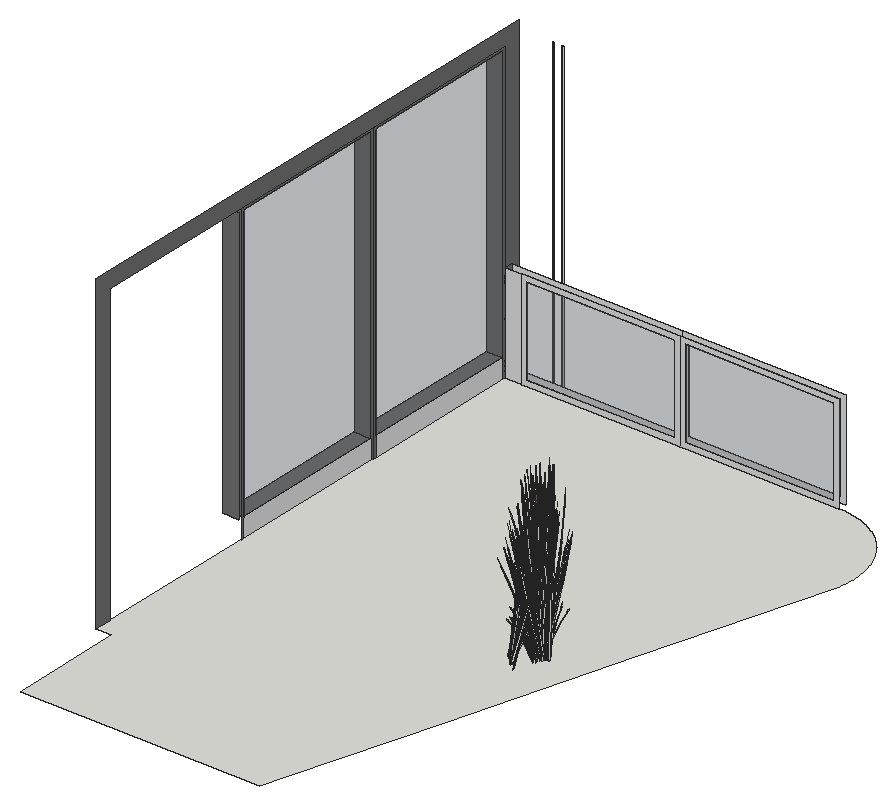
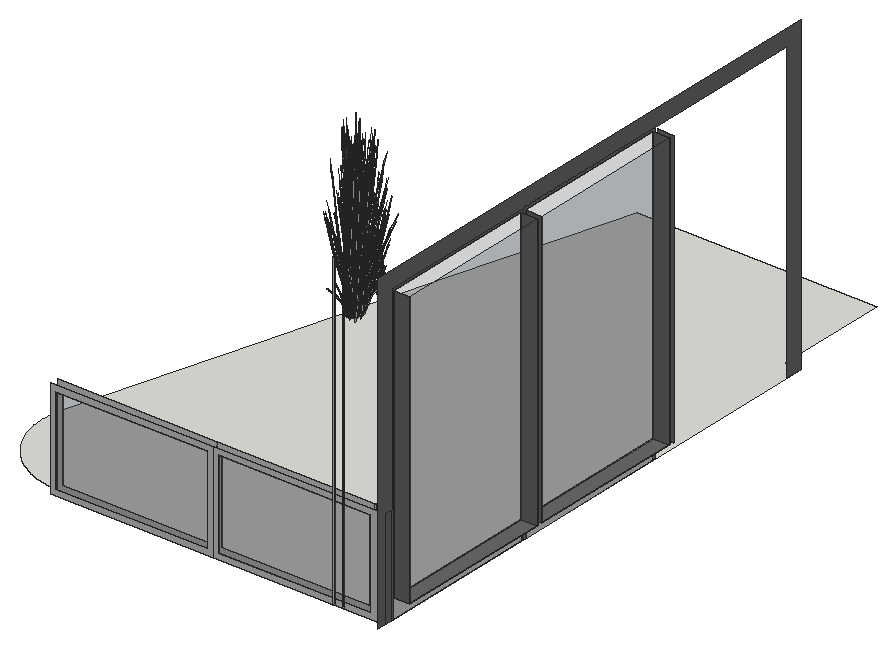
# SketchUp Ruby script. Lengths in inches.
U = 1.inch
M = Sketchup.active_model
def pt(a) = Geom::Point3d.new(a.map { |v| v * U })
def face(e, loops, mat)
  f = e.add_face(loops[0].map { |a| pt(a) })
  loops[1..].each { |l| e.add_face(l.map { |a| pt(a) }).erase! }
  f.material = f.back_material = mat if mat
  f
end
# faces: each face lists its corners as indices into pts; further lists are holes
def faces(e, pts, list, mat = nil) = list.each { |f| face(e, (f[0].is_a?(Array) ? f : [f]).map { |l| l.map { |i| pts[i] } }, mat) }
# xy, xz, yz: faces in a plane at the given z, y or x. An outline is a flat list of corners, or four numbers for a rectangle; further outlines are holes
def ring(l) = l.size == 4 ? [[l[0], l[1]], [l[2], l[1]], [l[2], l[3]], [l[0], l[3]]] : l.each_slice(2).to_a
def flat(e, list, mat, &to3) = list.each { |f| face(e, (f[0].is_a?(Array) ? f : [f]).map { |l| ring(l).map { |u, v| to3.(u, v) } }, mat) }
def xy(e, z, list, mat = nil) = flat(e, list, mat) { |x, y| [x, y, z] }
def xz(e, y, list, mat = nil) = flat(e, list, mat) { |x, z| [x, y, z] }
def yz(e, x, list, mat = nil) = flat(e, list, mat) { |y, z| [x, y, z] }
def lines(e, pts, list) = list.each { |a, b| e.add_line(pt(pts[a]), pt(pts[b])) }
# prism: a flat outline (further loops are holes) pulled along v
def prism(e, loops, v, mat = nil)
  f = face(e, loops, mat); d = Geom::Vector3d.new(v.map { |x| x * U })
  f.pushpull(f.normal.samedirection?(d) ? d.length : -d.length)
end
def box(e, o, s, mat = nil) = prism(e, [[o, [o[0] + s[0], o[1], o[2]], [o[0] + s[0], o[1] + s[1], o[2]], [o[0], o[1] + s[1], o[2]]]], [0, 0, s[2]], mat)
def at(x, y, z, deg = 0) = Geom::Transformation.translation(pt([x, y, z])) * Geom::Transformation.rotation(ORIGIN, Z_AXIS, deg.degrees)
def axes(o, x, y, z) = Geom::Transformation.new([*x, 0, *y, 0, *z, 0, *pt(o).to_a, 1])
def part(name) = M.definitions.add(name)
# library, detail: a bought-in or finely detailed component or shape, given as its bounding box
def library(name, o, s) = part(name).tap { |d| box(d.entities, o, s) }
def detail(e, o, s) = box(e.add_group.entities, o, s)
def put(e, d, t, mat = nil) = e.add_instance(d, t).tap { |i| i.material = mat if mat }
def group(e, t, mat = nil) = e.add_group.tap { |g| g.transformation = t; g.material = mat if mat }.entities
root = M.entities
M.materials.add("Glass_Basic_01").color = [105, 113, 122]
M.materials["Glass_Basic_01"].alpha = 0.25
M.materials.add("LightPink_Translucent").color = [144, 107, 117]
M.materials["LightPink_Translucent"].alpha = 0.75
M.materials.add("M01_Silver_Fog").color = [224, 224, 224]
M.materials.add("M06_Steel_Smoke").color = [114, 114, 114]
c1 = part("blade")
p = [[2.15,0.21,22],[0,0.17,0],[0.09,0.45,0],[2.18,0.31,22],[2.29,0.31,22],[0.38,0.45,0],
  [2.48,0.24,33],[2.49,0.24,33],[2.48,0.22,33]]
faces(c1.entities,p,[[0,1,2,3],[4,5,2,3],[6,3,4,7],[8,0,3,6]])
c2 = part("seeds")
p = [[0.3,-0.1,1.38],[-0.01,-0.03,1.59],[-0.01,-0.03,0.03],[0.14,-0.07,-0.07],[0.29,-0.03,3],[0.15,0.01,3.11]]
faces(c2.entities,p,[[0,1,2,3],[1,0,4,5]],"LightPink_Translucent")
c3 = part("blade with seeds")
put(c3.entities,c1,at(0,0,0))
put(c3.entities,c2,axes([2.4,0.25,30.99],[1.5799,-0.05474,1.17369],[-0.12525,1.92788,0.29478],[-0.07173,-0.02425,1.56792]))
xy(root,270,[[216,246,303.26,246,306,255.36,321.22,307.35,340.07,371.78,359.17,437.01,359.4,437.91,359.63,439,359.83,440.1,359.98,441.21,360.09,442.32,360.16,443.43,360.1875,444.55,360.17,445.67,360.11,446.78,360.01,447.89,359.87,449,359.68,450.1,359.45,451.2,359.18,452.28,358.875,453.35,358.52,454.41,358.13,455.46,357.7,456.49,357.23,457.5,356.73,458.5,356.18,459.47,355.6,460.43,354.98,461.36,354.33,462.26,353.64,463.14,352.92,464,352.17,464.83,351.39,465.62,350.58,466.39,349.74,467.125,348.87,467.83,347.97,468.5,347.05,469.13,346.11,469.73,345.15,470.29,344.16,470.82,343.16,471.3,342.13,471.75,341.09,472.16,340.04,472.53,338.97,472.86,337.89,473.15,336.8,473.4,335.71,473.6,334.6,473.77,333.49,473.89,332.38,473.97,331.45,474,210,474,210,288,213,288,213,287.79,216,287.79]])
xy(root,277,[[204,355,210,413],[204,415,210,473]],"M06_Steel_Smoke")
xz(root,353,[[204,277,210,377]],"M06_Steel_Smoke")
xz(root,355,[[204,277,210,377]],"M06_Steel_Smoke")
xz(root,413,[[204,277,210,377]],"M06_Steel_Smoke")
xz(root,415,[[204,277,210,377]],"M06_Steel_Smoke")
xz(root,473,[[204,277,210,377]],"M06_Steel_Smoke")
xz(root,474,[[218,272,271.49,304],[275.49,272,329.45,304]],"Glass_Basic_01")
xz(root,474,[[210,270,215.53,306],[215.53,270,216,306],[[216,270,273.49,306],[218,272,271.49,304]],[[273.49,270,331.45,306],[275.49,272,329.45,304]]],"M01_Silver_Fog")
xz(root,477,[[215,272,270.25,304],[274.25,272,329.5,304]],"Glass_Basic_01")
xz(root,477,[[[210,270,272.25,306],[215,272,270.25,304]],[[272.25,270,331.5,306],[274.25,272,329.5,304]]],"M01_Silver_Fog")
xz(root,477.03,[[225.03,270,225.12,383.24],[225.12,270,225.2,383.24],[225.2,270,225.29,383.24],[228.34,270,228.43,383.24],[228.43,270,228.52,383.24],
  [228.52,270,228.6,383.24]],"M01_Silver_Fog")
yz(root,204,[[355,277,413,377],[415,277,473,377]],"Glass_Basic_01")
yz(root,210,[[355,277,413,377],[415,277,473,377]],"Glass_Basic_01")
yz(root,210,[[355,270,413,277],[415,270,473,277]],"M01_Silver_Fog")
yz(root,210,[[288,270,294,270,294,378,474,378,474,306,477,306,477,270,480,270,480,384,288,384],[354,270,355,270,355,377,413,377,413,270,414,270,414,378,354,378],[414,270,415,270,415,377,473,377,473,270,474,270,474,378,414,378],[474,270,477,306]],"M06_Steel_Smoke")
p = [[224.94,477.04,270],[225.03,477.03,270],[225.03,477.03,383.24],[224.94,477.04,383.24],[224.85,477.06,270],[224.85,477.06,383.24],
  [225.29,477.03,270],[225.38,477.04,270],[225.38,477.04,383.24],[225.29,477.03,383.24],[228.17,477.06,270],[228.25,477.04,270],
  [228.25,477.04,383.24],[228.17,477.06,383.24],[228.34,477.03,270],[228.34,477.03,383.24],[228.6,477.03,270],[228.69,477.04,270],
  [228.69,477.04,383.24],[228.6,477.03,383.24]]
faces(root,p,[[0,1,2,3],[4,0,3,5],[6,7,8,9],[10,11,12,13],[11,14,15,12],[16,17,18,19]],"M01_Silver_Fog")
put(root,c3,axes([325.15,344.34,274.77],[0.06446,0.31404,1.1486],[-0.35756,-0.17393,0.84392],[0.03848,-0.1608,0.25299]))
put(root,c3,axes([320.96,338.65,273.49],[0.08132,-0.0293,1.76342],[0.48914,0.1613,-0.26939],[0.0143,0.18179,0.30037]))
put(root,c3,axes([323.96,344.07,276.71],[-0.00937,0.06455,1.77383],[-0.46231,0.23427,-0.16761],[-0.13604,-0.11975,0.31391]))
put(root,c3,axes([320.23,338.18,277],[0.35968,0.36185,-0.5672],[-0.37996,0.3169,-0.43934],[-0.05473,0.18385,1.08528]))
put(root,c3,axes([319.84,338.72,274.82],[0.45645,-0.09537,0.06507],[0.10494,0.38421,-0.86304],[-0.02894,0.19449,0.7736]))
put(root,c3,axes([321.3,338.53,276.68],[0.49392,0.135,-0.51099],[-0.1693,0.46287,-0.3958],[0.04529,0.18636,0.97773]))
put(root,c3,axes([321.58,337.57,275.875],[-0.11485,-0.17291,1.71376],[0.53072,-0.14557,0.13857],[0.11995,0.27145,0.73262]))
put(root,c3,axes([323.86,345.21,277.09],[0.55971,-0.13842,0.53763],[0.09714,0.54299,0.4433],[-0.13164,-0.16003,1.11249]))
put(root,c3,axes([325.13,345.3125,276.73],[0.4951,0.14079,0.48003],[-0.1693,0.46287,0.3958],[-0.02975,-0.18203,0.9933]))
put(root,c3,axes([325.27,345.48,277.03],[-0.49168,0.25073,-0.1216],[-0.24162,-0.44501,-0.67495],[-0.06487,-0.18753,1.02557]))
put(root,c3,axes([326.29,346.04,277.03],[-0.55221,-0.02668,-0.1216],[0.01509,-0.50521,-0.67495],[0.03836,-0.19458,1.02557]))
put(root,c3,axes([323.31,344.72,274.77],[0.2621,0.18744,1.1486],[-0.38171,0.11267,0.84392],[-0.08167,-0.14405,0.25299]))
put(root,c3,axes([321.07,338.8125,276.53],[-0.15148,0.41415,-0.35414],[-0.44193,-0.12079,0.4572],[0.04052,0.16674,0.87481]))
put(root,c3,axes([325.26,345.28,276.73],[0.37023,-0.18303,0.0643],[0.18122,0.33376,0.50621],[-0.03575,-0.14712,0.77189]))
put(root,c3,axes([323.95,345.71,276.98],[-0.42844,-0.2603,-0.71045],[0.30448,-0.45614,0.08574],[-0.15523,-0.15542,1.00501]))
put(root,c3,axes([323.8,345.37,276.53],[-0.0776,-0.43378,-0.35414],[0.44361,-0.11454,0.4572],[-0.11915,-0.12431,0.87481]))
put(root,c3,axes([320.12,338.01,277.34],[-0.01307,0.49815,-0.7886],[-0.55054,-0.03346,0.09517],[-0.0581,0.21104,1.11556]))
put(root,c3,axes([318.68,339.32,276.71],[0.057,-0.03251,1.77383],[0.47114,0.21627,-0.16761],[-0.01107,0.18007,0.31391]))
put(root,c3,axes([320.64,337.66,275.875],[-0.0123,-0.2067,1.71376],[0.53301,0.13712,0.13857],[-0.03297,0.29456,0.73262]))
put(root,c3,axes([323.99,345.33,276.73],[0.22836,-0.34211,0.0643],[0.3252,0.19918,0.50621],[-0.10513,-0.10968,0.77189]))
put(root,c3,axes([323.11,345.28,273.49],[-0.04867,0.07094,1.76342],[-0.49185,0.15296,-0.26939],[-0.11882,-0.13915,0.30037]))
put(root,c3,axes([321.12,338.44,276.98],[0.23981,0.43789,-0.71045],[-0.49365,0.24404,0.08574],[0.05608,0.21158,1.00501]))
put(root,c3,axes([323.92,347.23,274.1],[-0.20635,-0.55225,-0.69835],[0.59439,-0.19889,-0.18329],[-0.02281,-0.18701,1.54149]))
put(root,c3,axes([322.84,346,275.875],[0.18664,0.09279,1.71376],[-0.38624,0.38925,0.13857],[-0.24072,-0.1756,0.73262]))
put(root,c3,axes([319.73,339.13,274.59],[0.15856,-0.08496,1.43002],[0.39147,0.25616,-0.30754],[-0.11652,0.22165,0.61141]))
put(root,c3,axes([320.76,339.55,276.72],[0.06369,0.08672,1.74944],[0.51399,0.03407,-0.27667],[0.05169,0.19126,0.14031]))
put(root,c3,axes([325.12,345.65,277.05],[-0.15148,0.41415,0.35414],[-0.44193,-0.12079,-0.4572],[-0.04052,-0.16674,0.87481]))
put(root,c3,axes([323.75,345.73,276.68],[-0.4958,0.12802,-0.51099],[-0.08673,-0.48481,-0.3958],[-0.13317,-0.13893,0.97773]))
put(root,c3,axes([324.09,345.29,277.43],[-0.33533,0.51628,-0.13619],[-0.48563,-0.29744,-0.75594],[-0.16881,-0.14586,1.14864]))
put(root,c3,axes([323.84,345.65,274.375],[-0.31414,-0.53965,0],[0.52557,-0.30095,-0.51607],[0.1197,-0.06854,1.63711]))
put(root,c3,axes([324.53,345,274.13],[-0.34721,0.30895,-0.03893],[-0.31814,-0.33837,-0.17649],[-0.0224,-0.09588,0.58215]))
put(root,c3,axes([319.93,338.71,275.36],[0.01104,-0.27801,1.54345],[0.49652,0.14685,0.21329],[-0.04302,0.2963,0.72882]))
put(root,c3,axes([322.81,345.14,276.72],[-0.10811,-0.0038,1.74944],[-0.34418,0.38014,-0.27667],[-0.18364,-0.07767,0.14031]))
put(root,c3,axes([324.97,348.66,275.33],[0.4342,0.21716,1.51261],[-0.42537,0.46784,0.59816],[-0.19053,-0.27728,1.26806]))
put(root,c3,axes([324.0625,345.72,277.05],[0.0776,0.43378,0.35414],[-0.44361,0.11454,-0.4572],[-0.11915,-0.12431,0.87481]))
put(root,c3,axes([322.7,347.16,274.02],[0,-0.53854,-0.49651],[0.56215,0,0],[0,-0.12266,1.57504]))
put(root,c3,axes([322.73,346,277.09],[0.41494,-0.39744,0.53763],[0.35786,0.42207,0.4433],[-0.19468,-0.07331,1.11249]))
put(root,c3,axes([322.92,346,276.73],[0.0253,-0.40952,0.0643],[0.38204,0.01123,0.50621],[-0.14634,-0.04285,0.77189]))
put(root,c3,axes([324.23,347.375,274.21],[0.24378,-0.48527,-0.44739],[0.50654,0.23354,0.21531],[0,-0.11186,1.43643]))
put(root,c3,axes([322.77,346.13,276.53],[-0.28589,-0.33718,-0.35414],[0.32644,-0.31919,0.4572],[-0.16586,-0.04856,0.87481]))
put(root,c3,axes([322.94,347.17,274.03],[0.35073,-0.33601,-0.30978],[0.35073,0.33601,0.30978],[0,-0.10823,1.38974]))
put(root,c3,axes([322.8,345.56,274.13],[-0.14494,0.43975,-0.03893],[-0.4461,-0.13527,-0.17649],[-0.06773,-0.07192,0.58215]))
put(root,c3,axes([324.17,347.78,274.67],[-0.56585,-0.25696,-0.29095],[0.27246,-0.54236,-0.50002],[-0.01778,-0.13316,1.59708]))
put(root,c3,axes([322.5625,347.56,274.375],[-0.62828,0,0],[0,-0.6019,-0.51607],[0,-0.13709,1.63711]))
put(root,c3,axes([322.67,346.49,274.59],[0.0981,0.14994,1.43002],[-0.22605,0.40756,-0.30754],[-0.23211,-0.09741,0.61141]))
put(root,c3,axes([323.07,346.36,276.98],[-0.50227,-0.01297,-0.71045],[0.03373,-0.54602,0.08574],[-0.21278,-0.05762,1.00501]))
put(root,c3,axes([323.05,347.41,274.33],[-0.46736,0.45277,0.30756],[-0.46764,-0.44801,-0.36492],[-0.01632,-0.12858,1.64885]))
put(root,c3,axes([322.39,345.47,276.71],[0.03725,0.05374,1.77383],[-0.17957,0.48312,-0.16761],[-0.18186,0.0035,0.31391]))
put(root,c3,axes([324.53,347.62,274.43],[0.56613,0.26102,0.24065],[-0.27246,0.54236,0.50002],[0,-0.12502,1.60543]))
put(root,c3,axes([324.3125,348.35,274.4375],[0.13317,-0.63814,-0.23429],[0.63143,0.11124,0.51271],[-0.11033,-0.08813,1.5644]))
put(root,c3,axes([322.91,346.47,276.68],[-0.36484,0.35674,-0.51099],[-0.31952,-0.37685,-0.3958],[-0.18537,-0.05428,0.97773]))
put(root,c3,axes([323.18,346.31,277.05],[0.28589,0.33718,0.35414],[-0.32644,0.31919,-0.4572],[-0.16586,-0.04856,0.87481]))
put(root,c3,axes([322.09,346.9375,274.77],[0.32078,-0.03854,1.1486],[-0.20348,0.33954,0.84392],[-0.15852,-0.05093,0.25299]))
put(root,c3,axes([324.35,347.25,274.72],[-0.54562,0.03324,0.44739],[-0.04934,-0.55185,-0.21531],[0.09768,-0.05593,1.43643]))
put(root,c3,axes([323.1,346.09,277.03],[-0.0269,0.54769,-0.1216],[-0.50939,-0.01497,-0.67495],[-0.19618,-0.03804,1.02557]))
put(root,c3,axes([322.94,347.66,274.48],[0,0.53854,0.49651],[-0.56215,0,0],[0,-0.12266,1.57504]))
put(root,c3,axes([322.45,346.85,275.875],[0.20841,-0.0122,1.71376],[-0.13825,0.52864,0.13857],[-0.297,-0.0327,0.73262]))
put(root,c3,axes([324.27,348.09,274.21],[-0.30184,-0.45202,-0.44739],[0.45719,-0.31831,0.21531],[-0.09768,-0.05593,1.43643]))
put(root,c3,axes([324.33,347.45,274.36],[0.21845,0.6022,0.45755],[-0.62418,0.20941,0.17955],[0.00763,-0.11065,1.58856]))
put(root,c3,axes([324.22,347.93,274.72],[-0.24378,0.48527,0.44739],[-0.50654,-0.23354,-0.21531],[0,-0.11186,1.43643]))
put(root,c3,axes([325.12,347.5,274.21],[0,-0.62313,0],[0.62828,0,0],[0,0,1.79456]))
put(root,c3,axes([324,348.26,274.06],[-0.52267,-0.08829,-0.62353],[0.11029,-0.54463,-0.16365],[-0.15598,-0.06599,1.37633]))
put(root,c3,axes([324.82,347.11,274.36],[-0.4166,0.48873,0.45755],[-0.49494,-0.43142,0.17955],[0.10044,-0.04877,1.58856]))
put(root,c3,axes([325.28,347.99,274.3],[-0.46736,-0.46353,-0.06131],[0.46764,-0.46381,0],[-0.01632,-0.01619,1.75571]))
put(root,c3,axes([324.1,346.31,274.47],[-0.14515,0.53522,0.17642],[-0.53115,-0.15146,0.35086],[0.09175,-0.00261,1.60407]))
put(root,c3,axes([322.36,347.25,276.73],[0.14195,-0.49104,0.48003],[0.46669,0.16791,0.3958],[-0.18353,0.02951,0.9933]))
put(root,c3,axes([322.33,347.12,276.73],[-0.18454,-0.3672,0.0643],[0.33652,-0.17973,0.50621],[-0.14834,0.03546,0.77189]))
put(root,c3,axes([324.39,348.04,274.36],[0.63506,0.11347,0.45755],[-0.12924,0.64083,0.17955],[-0.09281,-0.06188,1.58856]))
put(root,c3,axes([322.32,347.49,273.49],[0.01274,0.08487,1.76342],[-0.25688,0.44323,-0.26939],[-0.18246,-0.02234,0.30037]))
put(root,c3,axes([323.44,349.09,274.03],[-0.11803,-0.46926,-0.30978],[0.46876,-0.13325,0.30978],[-0.0945,-0.05411,1.38974]))
put(root,c3,axes([324.05,349.07,274.47],[0.53992,-0.14294,0.17642],[0.13332,0.53195,0.35086],[-0.04815,-0.07751,1.60407]))
put(root,c3,axes([323.3125,349.29,274.02],[-0.47024,-0.26927,-0.49651],[0.28107,-0.48284,0],[-0.1071,-0.06133,1.57504]))
put(root,c3,axes([322.27,347.3,276.53],[-0.41757,-0.15024,-0.35414],[0.12179,-0.4383,0.4572],[-0.16812,0.04019,0.87481]))
put(root,c3,axes([324.59,348.34,274.67],[-0.5073,0.35754,-0.29095],[-0.33735,-0.5052,-0.50002],[-0.12516,-0.05131,1.59708]))
put(root,c3,axes([325.7,346.34,274.47],[-0.53992,0.14294,0.17642],[-0.13332,-0.53195,0.35086],[0.04815,0.07751,1.60407]))
put(root,c3,axes([325.36,347.36,274.38],[-0.63506,-0.11347,0.49198],[0.12924,-0.64083,0.19306],[0.09281,0.06188,1.70813]))
put(root,c3,axes([324.86,348.94,274.2],[-0.16394,-0.4643,0],[0.46814,-0.1626,0],[0,0,1.54371]))
put(root,c3,axes([324.54,348.5,274.62],[-0.09693,0.48062,0.1448],[-0.47357,-0.08343,-0.41347],[-0.08619,-0.04935,1.26744]))
put(root,c3,axes([322.71,347.25,277.05],[0.41757,0.15024,0.35414],[-0.12179,0.4383,-0.4572],[-0.16812,0.04019,0.87481]))
put(root,c3,axes([325.65,349.1,274.47],[0.14515,-0.53522,0.17642],[0.53115,0.15146,0.35086],[-0.09175,0.00261,1.60407]))
put(root,c3,axes([325.53,347.88,274.21],[0.35073,0.34786,0],[-0.35073,0.34786,0],[0,0,1.69266]))
put(root,c3,axes([323.54,347.23,275.34],[0.14282,-0.0779,1.77064],[0.04925,0.54394,0.13857],[-0.30935,0.07218,0.63284]))
put(root,c3,axes([326.48,347.73,274.47],[-0.39477,-0.39228,0.17642],[0.39783,-0.38049,0.35086],[-0.0436,0.08011,1.60407]))
put(root,c3,axes([324.74,349.15,274.2],[-0.50654,-0.24178,0],[0.24378,-0.50239,0],[0,0,1.62707]))
put(root,c3,axes([325.16,348.51,274.46],[-0.49063,-0.43346,-0.25192],[0.41285,-0.48673,0.5513],[-0.13212,0.05071,1.68216]))
put(root,c3,axes([323.87,349.34,274.48],[0.47024,0.26927,0.49651],[-0.28107,0.48284,0],[-0.1071,-0.06133,1.57504]))
put(root,c3,axes([325.53,347.47,274.72],[0.24378,-0.48527,0.44739],[0.50654,0.23354,-0.21531],[0,0.11186,1.43643]))
put(root,c3,axes([322,347.59,276.72],[-0.08205,0.06992,1.74944],[0.00698,0.51086,-0.27667],[-0.18807,0.06644,0.14031]))
put(root,c3,axes([325.43,347.75,274.29],[0,0.62282,-0.05637],[-0.62828,0,0],[0,0.01957,1.79368]))
put(root,c3,axes([322.55,347.52,276.68],[-0.13612,0.48987,-0.51099],[-0.46669,-0.16791,-0.3958],[-0.1879,0.04492,0.97773]))
put(root,c3,axes([322.53,347.11,277.03],[0.25281,0.48765,-0.1216],[-0.44869,0.23964,-0.67495],[-0.18908,0.06434,1.02557]))
put(root,c3,axes([323.6,349.62,274.375],[-0.31414,0.53965,0],[-0.52557,-0.30095,-0.51607],[-0.1197,-0.06854,1.63711]))
put(root,c3,axes([325.4,348.15,274.72],[0.54562,-0.03324,0.44739],[0.04934,0.55185,-0.21531],[-0.09768,0.05593,1.43643]))
put(root,c3,axes([324.91,348.42,274.21],[-0.54562,0.03324,-0.44739],[-0.04934,-0.55185,0.21531],[-0.09768,0.05593,1.43643]))
put(root,c3,axes([325.32,349.16,274.2],[0.50654,0.24178,0],[-0.24378,0.50239,0],[0,0,1.74954]))
put(root,c3,axes([325.52,349.69,274.19],[-0.31023,-0.54153,-0.05142],[0.52557,-0.30095,0.51607],[-0.12951,0.05156,1.6363]))
put(root,c3,axes([325.41,348.39,274.62],[0.37121,0.32357,0.1448],[-0.30963,0.36505,-0.41347],[-0.08619,0.04935,1.26744]))
put(root,c3,axes([322.48,348.47,276.73],[-0.12461,-0.49565,0.48003],[0.48882,-0.08602,0.3958],[-0.14406,0.11657,0.9933]))
put(root,c3,axes([322.38,348.375,276.73],[-0.34493,-0.22649,0.0643],[0.20082,-0.32253,0.50621],[-0.11059,0.10427,0.77189]))
put(root,c3,axes([322.54,347.78,275.875],[0.17434,-0.11391,1.71376],[0.14677,0.52637,0.13857],[-0.27369,0.11897,0.73262]))
put(root,c3,axes([325.8,349.38,274.48],[0.47024,-0.26927,0.49651],[0.28107,0.48284,0],[-0.1071,0.06133,1.57504]))
put(root,c3,axes([325.13,348.96,274.29],[0.21845,0.61869,-0.06012],[-0.62418,0.21679,0],[0.00763,0.02161,1.72173]))
put(root,c3,axes([325.375,349.625,274.03],[-0.46876,-0.13325,-0.30978],[0.11803,-0.46926,0.30978],[-0.0945,0.05411,1.38974]))
put(root,c3,axes([321.99,348.67,274.59],[0.17462,0.04421,1.43002],[0.11254,0.45156,-0.30754],[-0.23719,0.08453,0.61141]))
put(root,c3,axes([322.78,348.31,277.05],[0.43736,-0.07697,0.35414],[0.11549,0.43998,-0.4572],[-0.12533,0.11818,0.87481]))
put(root,c3,axes([321.09,348.11,276.71],[0.06412,0.01444,1.77383],[0.19837,0.47583,-0.16761],[-0.13126,0.12489,0.31391]))
put(root,c3,axes([326.9375,348.15,274.2],[-0.62797,-0.00431,-0.04976],[0,-0.6019,0.49943],[-0.01973,0.13702,1.58352]))
put(root,c3,axes([321.63,349.62,274.77],[0.2094,-0.24408,1.1486],[0.08263,0.38639,0.84392],[-0.15132,0.06919,0.25299]))
put(root,c3,axes([326.81,348.23,274.03],[-0.35073,0.33601,-0.30978],[-0.35073,-0.33601,0.30978],[0,0.10823,1.38974]))
put(root,c3,axes([325.3,348.27,274.67],[0.05855,0.61451,-0.29095],[-0.60981,0.03716,-0.50002],[-0.10738,0.08185,1.59708]))
put(root,c3,axes([325.52,348.03,274.21],[-0.24378,0.48527,-0.44739],[-0.50654,-0.23354,0.21531],[0,0.11186,1.43643]))
put(root,c3,axes([322.42,348.57,276.53],[-0.43736,0.07697,-0.35414],[-0.11549,-0.43998,0.4572],[-0.12533,0.11818,0.87481]))
put(root,c3,axes([321.78,349.55,277.65],[0.44338,0.14375,-0.06488],[-0.13639,0.44245,-0.29416],[-0.07252,0.06718,0.97024]))
put(root,c3,axes([324.93,348.73,274.06],[-0.33843,0.40479,-0.62353],[-0.42041,-0.36705,-0.16365],[-0.13561,0.10098,1.37633]))
put(root,c3,axes([325.53,349.42,274.33],[0.62903,0.17504,0.30756],[-0.15737,0.62568,-0.36492],[-0.10411,0.07831,1.64885]))
put(root,c3,axes([325.49,349.84,274.02],[-0.47024,0.26927,-0.49651],[-0.28107,-0.48284,0],[-0.1071,0.06133,1.57504]))
put(root,c3,axes([322.55,348.26,277.03],[0.46478,0.29695,-0.1216],[-0.26776,0.43004,-0.67495],[-0.13131,0.14949,1.02557]))
put(root,c3,axes([323.18,348.13,275.875],[0.1255,-0.16547,1.71376],[0.31687,0.44665,0.13857],[-0.21734,0.2034,0.73262]))
put(root,c3,axes([322.78,348.62,276.68],[0.12908,0.49174,-0.51099],[-0.48882,0.08602,-0.3958],[-0.14008,0.13208,0.97773]))
put(root,c3,axes([323.37,349.18,277.05],[0.33997,-0.28354,0.35414],[0.32182,0.32376,-0.4572],[-0.04897,0.1645,0.87481]))
put(root,c3,axes([325.91,349.76,274.375],[0.31414,0.53965,0],[-0.52557,0.30095,-0.51607],[-0.1197,0.06854,1.63711]))
put(root,c3,axes([325.65,347.62,274.84],[-0.01373,-0.50706,1.41272],[0.62119,0.13144,0.59816],[-0.14692,0.27746,1.3335]))
put(root,c3,axes([325.81,348.17,274.09],[0.18424,0.49308,-0.69212],[-0.53071,0.17758,-0.18165],[0.02036,0.16697,1.52773]))
put(root,c3,axes([323.06,349.4375,276.73],[-0.4129,-0.02509,0.0643],[0.01132,-0.37891,0.50621],[-0.04321,0.14514,0.77189]))
put(root,c3,axes([322.18,349.87,273.49],[0.0674,0.0538,1.76342],[0.11428,0.49852,-0.26939],[-0.14937,0.10631,0.30037]))
put(root,c3,axes([323.19,349.47,276.73],[-0.35779,-0.36745,0.48003],[0.37996,-0.3169,0.3958],[-0.066,0.17239,0.9933]))
put(root,c3,axes([324.32,349.65,277.05],[0.15148,-0.41415,0.35414],[0.44193,0.12079,-0.4572],[0.04052,0.16674,0.87481]))
put(root,c3,axes([324.91,351.125,277.65],[0.34721,-0.30895,-0.06488],[0.31814,0.33837,-0.29416],[0.0224,0.09588,0.97024]))
put(root,c3,axes([323.08,348.54,275.875],[0.09355,-0.18511,1.71376],[0.39247,0.38307,0.13857],[-0.17705,0.23875,0.73262]))
put(root,c3,axes([324.18,350.02,276.73],[-0.37023,0.18303,0.0643],[-0.18122,-0.33376,0.50621],[0.03575,0.14712,0.77189]))
put(root,c3,axes([323.1875,349.58,276.53],[-0.33997,0.28354,-0.35414],[-0.32182,-0.32376,0.4572],[-0.04897,0.1645,0.87481]))
put(root,c3,axes([322.02,349.5,276.72],[-0.01249,0.10657,1.74944],[0.35444,0.37075,-0.27667],[-0.09279,0.17532,0.14031]))
put(root,c3,axes([323.15,349.26,277.4],[0.55221,0.02668,-0.13498],[-0.01509,0.50521,-0.74919],[-0.03836,0.19458,1.13838]))
put(root,c3,axes([324.17,349.82,277.03],[0.49168,-0.25073,-0.1216],[0.24162,0.44501,-0.67495],[0.06487,0.18753,1.02557]))
put(root,c3,axes([324.3125,349.99,277.0625],[-0.4951,-0.14079,0.53283],[0.1693,-0.46287,0.43934],[0.02975,0.18203,1.10256]))
put(root,c3,axes([323.41,350.69,274.77],[-0.013,-0.32022,1.1486],[0.32493,0.22839,0.84392],[-0.0639,0.15263,0.25299]))
put(root,c3,axes([324.26,349.92,273.49],[0.08132,-0.0293,1.76342],[0.48914,0.1613,-0.26939],[0.0143,0.18179,0.30037]))
put(root,c3,axes([323.53,349.45,277],[0.35968,0.36185,-0.5672],[-0.37996,0.3169,-0.43934],[-0.05473,0.18385,1.08528]))
put(root,c3,axes([323.14,349.99,274.82],[0.45645,-0.09537,0.06507],[0.10494,0.38421,-0.86304],[-0.02894,0.19449,0.7736]))
put(root,c3,axes([324.59,349.8,276.68],[0.49392,0.135,-0.51099],[-0.1693,0.46287,-0.3958],[0.04529,0.18636,0.97773]))
put(root,c3,axes([324.37,350.08,276.53],[-0.15148,0.41415,-0.35414],[-0.44193,-0.12079,0.4572],[0.04052,0.16674,0.87481]))
put(root,c3,axes([323.42,349.28,277.34],[-0.01307,0.49815,-0.7886],[-0.55054,-0.03346,0.09517],[-0.0581,0.21104,1.11556]))
put(root,c3,axes([321.98,350.59,276.71],[0.057,-0.03251,1.77383],[0.47114,0.21627,-0.16761],[-0.01107,0.18007,0.31391]))
put(root,c3,axes([323.9375,348.93,275.875],[-0.0123,-0.2067,1.71376],[0.53301,0.13712,0.13857],[-0.03297,0.29456,0.73262]))
put(root,c3,axes([324.41,349.71,276.98],[0.23981,0.43789,-0.71045],[-0.49365,0.24404,0.08574],[0.05608,0.21158,1.00501]))
put(root,c3,axes([323.03,350.4,274.59],[0.15856,-0.08496,1.43002],[0.39147,0.25616,-0.30754],[-0.11652,0.22165,0.61141]))
put(root,c3,axes([324.06,350.82,276.72],[0.06369,0.08672,1.74944],[0.51399,0.03407,-0.27667],[0.05169,0.19126,0.14031]))
put(root,c3,axes([323.23,349.99,275.36],[0.01104,-0.27801,1.54345],[0.49652,0.14685,0.21329],[-0.04302,0.2963,0.72882]))
